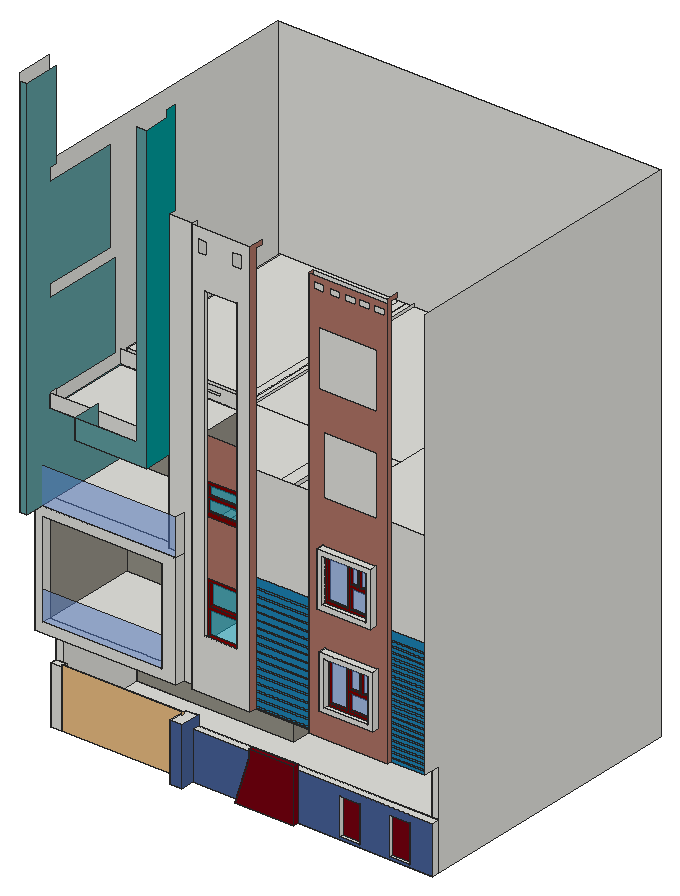
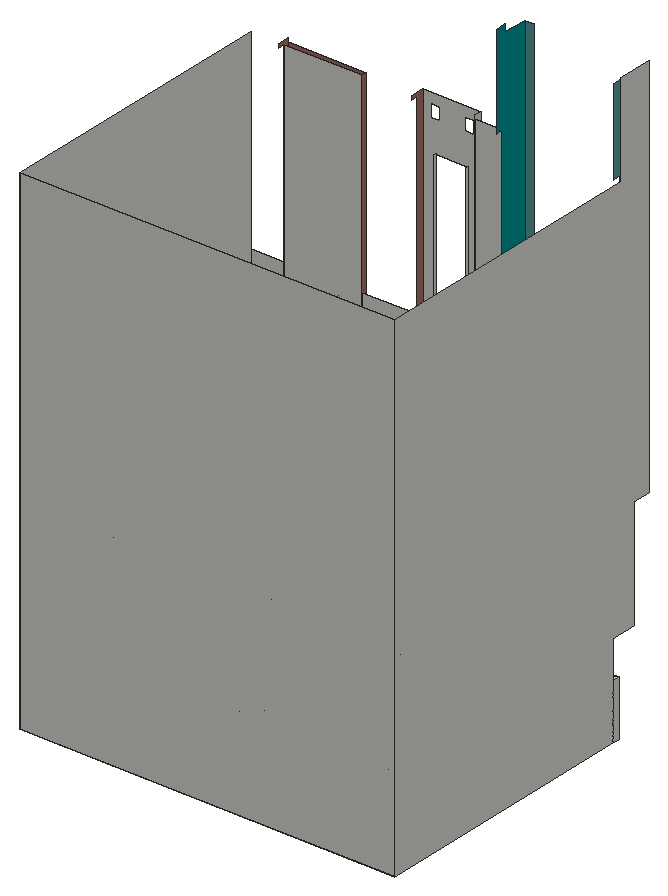
# SketchUp Ruby script. Lengths in inches.
U = 1.inch
M = Sketchup.active_model
def pt(a) = Geom::Point3d.new(a.map { |v| v * U })
def face(e, loops, mat)
  f = e.add_face(loops[0].map { |a| pt(a) })
  loops[1..].each { |l| e.add_face(l.map { |a| pt(a) }).erase! }
  f.material = f.back_material = mat if mat
  f
end
# faces: each face lists its corners as indices into pts; further lists are holes
def faces(e, pts, list, mat = nil) = list.each { |f| face(e, (f[0].is_a?(Array) ? f : [f]).map { |l| l.map { |i| pts[i] } }, mat) }
# xy, xz, yz: faces in a plane at the given z, y or x. An outline is a flat list of corners, or four numbers for a rectangle; further outlines are holes
def ring(l) = l.size == 4 ? [[l[0], l[1]], [l[2], l[1]], [l[2], l[3]], [l[0], l[3]]] : l.each_slice(2).to_a
def flat(e, list, mat, &to3) = list.each { |f| face(e, (f[0].is_a?(Array) ? f : [f]).map { |l| ring(l).map { |u, v| to3.(u, v) } }, mat) }
def xy(e, z, list, mat = nil) = flat(e, list, mat) { |x, y| [x, y, z] }
def xz(e, y, list, mat = nil) = flat(e, list, mat) { |x, z| [x, y, z] }
def yz(e, x, list, mat = nil) = flat(e, list, mat) { |y, z| [x, y, z] }
def lines(e, pts, list) = list.each { |a, b| e.add_line(pt(pts[a]), pt(pts[b])) }
# prism: a flat outline (further loops are holes) pulled along v
def prism(e, loops, v, mat = nil)
  f = face(e, loops, mat); d = Geom::Vector3d.new(v.map { |x| x * U })
  f.pushpull(f.normal.samedirection?(d) ? d.length : -d.length)
end
def box(e, o, s, mat = nil) = prism(e, [[o, [o[0] + s[0], o[1], o[2]], [o[0] + s[0], o[1] + s[1], o[2]], [o[0], o[1] + s[1], o[2]]]], [0, 0, s[2]], mat)
def at(x, y, z, deg = 0) = Geom::Transformation.translation(pt([x, y, z])) * Geom::Transformation.rotation(ORIGIN, Z_AXIS, deg.degrees)
def axes(o, x, y, z) = Geom::Transformation.new([*x, 0, *y, 0, *z, 0, *pt(o).to_a, 1])
def part(name) = M.definitions.add(name)
# library, detail: a bought-in or finely detailed component or shape, given as its bounding box
def library(name, o, s) = part(name).tap { |d| box(d.entities, o, s) }
def detail(e, o, s) = box(e.add_group.entities, o, s)
def put(e, d, t, mat = nil) = e.add_instance(d, t).tap { |i| i.material = mat if mat }
def group(e, t, mat = nil) = e.add_group.tap { |g| g.transformation = t; g.material = mat if mat }.entities
root = M.entities
M.materials.add("[0022_Maroon]").color = [128, 0, 0]
M.materials.add("[0081_CadetBlue]").color = [95, 158, 160]
M.materials.add("[0100_SteelBlue]").color = [29, 130, 180]
M.materials.add("[Color H07]").color = [0, 153, 153]
M.materials.add("[Formica Blue]").color = [71, 97, 152]
M.materials.add("[Formica Graystone]").color = [149, 146, 135]
M.materials.add("[Sketchy Siding Straight]").color = [119, 0, 16]
M.materials.add("[Stone Flagstone Ashlar]").color = [175, 116, 102]
M.materials.add("[Translucent Glass Blue]").color = [100, 149, 237]
M.materials["[Translucent Glass Blue]"].alpha = 0.5
M.materials.add("[Translucent Glass Tinted]").color = [8, 201, 241]
M.materials["[Translucent Glass Tinted]"].alpha = 0.48
c1 = library("gate (1)",[0,0,0],[171.26,1.97,78.74])
box(root,[9,163.25,173.75],[154.01,236.0625,120])
xy(root,41.75,[[164.3,31.6875,164.3,57.3125,360,57.3125,360,48.3125,312.21,48.3125,312.21,42.3125,238.26,42.3125,238.26,48.3125,179.85,48.3125,179.85,31.6875],[0,48.3125,13.95,57.3125],[360,48.3125,483.5625,57.3125],[0,57.3125,0,408.3125,360,408.3125,360,399.3125,9,399.3125,9,57.3125],[9,57.3125,474.5625,57.3125,474.5625,399.3125,207.375,399.3125,207.375,173.875,9,173.875],
  [474.5625,57.3125,474.5625,399.3125,360,399.3125,360,408.3125,483.5625,408.3125,483.5625,57.3125],[9,173.875,9,179.875,201.375,179.875,201.375,399.3125,207.375,399.3125,207.375,173.875],[9,179.875,201.375,399.3125]])
xy(root,44.78,[[365.45,48.3125,391.2,53],[428.88,48.3125,454.63,52.0625]])
xy(root,77.84,[[79.99,170.875,183.74,173.875]])
xy(root,78.43,[[21.52,170.875,59.52,173.875]])
xy(root,80.84,[[82.99,170.875,102.77,173.875],[106.875,170.875,180.74,173.875]],"[0022_Maroon]")
xy(root,81.43,[[24.52,170.875,56.52,173.875]],"[0022_Maroon]")
xy(root,91.78,[[365.45,48.3125,391.2,53],[428.88,48.3125,454.63,52.0625]])
xy(root,101.75,[[179.85,48.3125,483.5625,57.3125]])
xy(root,108.53,[[255.96,42.3125,312.21,48.3125]],"[Sketchy Siding Straight]")
xy(root,113.75,[[164.3,31.6875,179.85,57.3125],[0,48.3125,13.95,57.3125]])
xy(root,145.3,[[24.52,170.875,56.52,173.875]],"[0022_Maroon]")
xy(root,148.09,[[82.99,170.875,102.77,173.875],[106.875,170.875,180.74,173.875]],"[0022_Maroon]")
xy(root,148.3,[[21.52,170.875,59.52,173.875]])
xy(root,151.09,[[79.99,170.875,183.74,173.875]],"[0022_Maroon]")
xy(root,161.75,[[0,24,177.9375,36],[195.16,27,195.16,36,9,36,9,173.875,207.375,173.875,207.375,399.3125,474.5625,399.3125,474.5625,57.3125,483.5625,57.3125,483.5625,36,269.35,36,269.35,27],[341.01,30,440.77,36],[0,36,9,57.3125],[9,173.875,207.375,173.875,207.375,399.3125,201.375,399.3125,201.375,179.875,9,179.875],
  [9,179.875,201.375,399.3125]])
xy(root,173.75,[[9,24,160.01,36],[9,36,160.01,36,160.01,157.25,141.2,157.25,141.2,154.25,138.2,154.25,138.2,157.25,102.2,157.25,102.2,154.25,99.2,154.25,99.2,157.25,9,157.25],[99.2,154.25,102.2,157.25],[138.2,154.25,141.2,157.25]])
xy(root,197.9375,[[361.52,21,428.89,30]])
xy(root,203.9375,[[367.52,21,422.89,27]])
xy(root,206.9375,[[370.52,27,391.89,30],[395.21,27,419.89,30]],"[0022_Maroon]")
xy(root,218.125,[[18.2,154.25,89.13,157.25]])
xy(root,224.125,[[24.2,154.25,53.67,157.25],[57.96,154.25,83.13,157.25]],"[0022_Maroon]")
xy(root,227.89,[[395.21,27,419.89,30]],"[0022_Maroon]")
xy(root,228.47,[[211.91,27,253.16,27,253.16,30,250.36,30,250.36,32.1875,215.48,32.1875,215.48,30,211.91,30]],"[0022_Maroon]")
xy(root,231.625,[[395.21,27,407.55,30],[410.96,27,419.89,30]],"[0022_Maroon]")
xy(root,254.1875,[[57.96,154.25,83.13,157.25]],"[0022_Maroon]")
xy(root,256.3125,[[370.52,27,391.89,30],[395.21,27,407.55,30],[410.96,27,419.89,30]],"[0022_Maroon]")
xy(root,257.06,[[215.48,30,250.36,32.1875]],"[0022_Maroon]")
xy(root,257.75,[[102.2,154.25,138.2,157.25]],"[0022_Maroon]")
xy(root,259.3125,[[367.52,21,422.89,27]])
xy(root,259.36,[[57.96,154.25,83.13,157.25]],"[0022_Maroon]")
xy(root,260.75,[[99.2,154.25,141.2,157.25]],"[0022_Maroon]")
xy(root,261.21,[[215.48,30,250.36,35.4375]],"[0022_Maroon]")
xy(root,265.3125,[[361.52,21,428.89,30]])
xy(root,278.4375,[[24.2,154.25,53.67,157.25],[57.96,154.25,83.13,157.25]],"[0022_Maroon]")
xy(root,284.4375,[[18.2,154.25,89.13,157.25]],"[0022_Maroon]")
xy(root,289.07,[[215.48,30,250.36,35.4375]],"[0022_Maroon]")
xy(root,290.0625,[[9,36,160.01,157.25]],"[Formica Graystone]")
xy(root,293.75,[[9,24,160.01,36],[169.01,157.25,351,399.3125]])
xy(root,305.75,[[0,0,9,24],[9,23.22,9,24,177.9375,24],[9,24,177.9375,24,177.9375,36,160.01,36,160.01,45,9,45],[9,45,160.01,45,160.01,148.25,145.29,148.25,145.29,145.25,142.29,145.25,142.29,148.25,106.29,148.25,106.29,145.25,103.29,145.25,103.29,148.25,9,148.25],[103.29,145.25,106.29,148.25],
  [142.29,145.25,145.29,148.25],[160.01,148.25,169.01,157.25],[9,157.25,160.01,399.3125]])
xy(root,313.15,[[358.5,21,426.4375,30]])
xy(root,319.15,[[364.5,21,420.4375,27],[364.5,27,420.4375,30]])
xy(root,322.15,[[392.47,27,396.32,30]])
xy(root,322.15,[[367.5,27,392.47,30],[396.32,27,417.4375,30]],"[0022_Maroon]")
xy(root,337,[[25.5,145.25,96.62,148.25]])
xy(root,343,[[31.5,145.25,61.06,148.25],[64.41,145.25,90.62,148.25]],"[0022_Maroon]")
xy(root,347.12,[[396.32,27,417.4375,30]])
xy(root,350.93,[[396.32,27,405.07,30],[408.78,27,417.4375,30]],"[0022_Maroon]")
xy(root,368.85,[[214.81,30,250.11,31.875]],"[0022_Maroon]")
xy(root,372.09,[[367.5,27,392.47,30],[396.32,27,405.07,30],[408.78,27,417.4375,30]],"[0022_Maroon]")
xy(root,375.09,[[364.5,21,420.4375,27],[364.5,27,420.4375,30]])
xy(root,381.09,[[358.5,21,426.4375,30]])
xy(root,382.74,[[214.81,30,250.11,31.875]],"[0022_Maroon]")
xy(root,382.88,[[64.41,145.25,90.62,148.25]],"[0022_Maroon]")
xy(root,385.95,[[64.41,145.25,90.62,148.25]],"[0022_Maroon]")
xy(root,386.41,[[214.81,30,250.11,32.875]],"[0022_Maroon]")
xy(root,389.75,[[106.29,145.25,142.29,148.25]],"[0022_Maroon]")
xy(root,392.75,[[103.29,145.25,145.29,148.25]],"[0022_Maroon]")
xy(root,399,[[31.5,145.25,61.06,148.25],[64.41,145.25,90.62,148.25]],"[0022_Maroon]")
xy(root,399.35,[[214.81,30,250.11,32.875]])
xy(root,405,[[25.5,145.25,96.62,148.25]],"[0022_Maroon]")
xy(root,411.4375,[[9,36,160.01,148.25]])
xy(root,411.4375,[[69.02,0,160.01,36]],"[0081_CadetBlue]")
xy(root,425.75,[[160.01,148.25,169.01,157.25],[169.01,148.25,170.26,399.3125],[170.26,148.25,178.01,399.3125],[178.01,148.25,363.3125,399.3125],[9,157.25,160.01,399.3125],
  [160.01,157.25,169.01,399.3125]])
xz(root,0,[[0,305.75,9,794.55],[69.02,411.4375,160.01,411.4375,160.01,794.55,148.21,794.55,148.21,437.26,69.02,437.26]],"[0081_CadetBlue]")
xz(root,21,[[[361.52,197.9375,428.89,265.3125],[367.52,203.9375,422.89,259.3125]],[[358.5,313.15,426.4375,381.09],[364.5,319.15,420.4375,375.09]]])
xz(root,24,[[[0,161.75,177.9375,305.75],[9,173.75,160.01,293.75]]])
xz(root,24,[[9,173.75,160.01,211.88]],"[Translucent Glass Blue]")
xz(root,27,[[[195.16,161.75,269.35,688.75],[211.91,228.47,253.16,619.47],[203.22,659.36,215.03,675.93],[246.9,659.36,258.72,675.93]]])
xz(root,27,[[[367.52,203.9375,422.89,259.3125],[370.52,206.9375,391.89,256.3125],[395.21,206.9375,419.89,227.89],[395.21,231.625,407.55,256.3125],[410.96,231.625,419.89,256.3125]],[[364.5,319.15,420.4375,375.09],[367.5,322.15,367.5,372.09,392.47,372.09,392.47,322.15,396.32,322.15,396.32,347.12,417.4375,347.12,417.4375,322.15],[396.32,350.93,405.07,372.09],[408.78,350.93,417.4375,372.09]]],"[0022_Maroon]")
xz(root,30,[[[364.5,319.15,420.4375,375.09],[367.5,322.15,417.4375,322.15,417.4375,347.12,396.32,347.12,396.32,322.15,392.47,322.15,392.47,372.09,367.5,372.09],[396.32,350.93,405.07,372.09],[408.78,350.93,417.4375,372.09]]])
xz(root,30,[[[211.91,228.47,215.48,228.47,215.48,257.06,250.36,257.06,250.36,228.47,253.16,228.47,253.16,292.67,211.91,292.67],[215.48,261.21,250.36,289.07]],[[211.91,362.68,253.16,402.99],[214.81,368.85,250.11,382.74],[214.81,386.41,250.11,399.35]]],"[0022_Maroon]")
xz(root,30,[[[341.01,161.75,440.77,683.75],[353.5625,556.6,427.4375,626.6],[359.73,434.83,427.1,510.21],[358.5,313.15,426.4375,381.09],[361.52,197.9375,428.89,265.3125],[347.12,668.19,360.37,676.37],[367.68,668.19,380.93,676.37],[387.06,668.19,400.31,676.37],[404.68,668.19,417.93,676.37],[423.62,668.19,436.87,676.37]],[211.91,292.67,253.16,362.68],[211.91,402.99,253.16,454.38]],"[Stone Flagstone Ashlar]")
xz(root,30,[[370.52,206.9375,391.89,256.3125],[395.21,206.9375,419.89,227.89],[395.21,231.625,407.55,256.3125],[410.96,231.625,419.89,256.3125],[367.5,322.15,392.47,372.09],
  [396.32,322.15,417.4375,347.12],[396.32,350.93,405.07,372.09],[408.78,350.93,417.4375,372.09]],"[Translucent Glass Blue]")
xz(root,31.6875,[[164.3,41.75,179.85,113.75]],"[Formica Blue]")
xz(root,31.875,[[214.81,368.85,250.11,382.74]],"[Translucent Glass Tinted]")
xz(root,32.1875,[[215.48,228.47,250.36,257.06]],"[Translucent Glass Tinted]")
xz(root,32.875,[[214.81,386.41,250.11,399.35]],"[Translucent Glass Tinted]")
xz(root,35.4375,[[215.48,261.21,250.36,289.07]],"[Translucent Glass Tinted]")
xz(root,36,[[177.9375,161.75,195.16,161.75,195.16,683.75,160.01,683.75,160.01,305.75,177.9375,305.75],[341.01,161.75,440.77,683.75],[160.01,173.75,177.9375,293.375],[9,290.0625,160.01,293.375],[9,293.375,160.01,293.75],
  [269.35,311.26,341.01,432.69],[440.77,311.26,483.5625,433.25],[9,411.4375,69.02,428.75],[69.02,411.4375,160.01,428.75]])
xz(root,36,[[269.35,161.75,341.01,163.11],[440.77,161.75,483.5625,165.93],[269.35,163.11,341.01,165.14],[269.35,165.14,341.01,172.11],[440.77,165.93,483.5625,168.01],
  [440.77,168.01,483.5625,172.55],[269.35,172.11,341.01,174.14],[440.77,172.55,483.5625,174.63],[269.35,174.14,341.01,181.11],[440.77,174.63,483.5625,179.18],
  [440.77,179.18,483.5625,181.26],[269.35,181.11,341.01,183.14],[440.77,181.26,483.5625,185.8],[269.35,183.14,341.01,190.11],[440.77,185.8,483.5625,187.88],
  [440.77,187.88,483.5625,192.43],[269.35,190.11,341.01,192.14],[269.35,192.14,341.01,199.11],[440.77,192.43,483.5625,194.51],[440.77,194.51,483.5625,199.05],
  [440.77,199.05,483.5625,201.13],[269.35,199.11,341.01,201.14],[440.77,201.13,483.5625,205.68],[269.35,201.14,341.01,208.11],[440.77,205.68,483.5625,207.76],
  [440.77,207.76,483.5625,212.3],[269.35,208.11,341.01,210.14],[269.35,210.14,341.01,217.11],[440.77,212.3,483.5625,214.38],[440.77,214.38,483.5625,218.93],
  [269.35,217.11,341.01,219.14],[440.77,218.93,483.5625,221.01],[269.35,219.14,341.01,226.11],[440.77,221.01,483.5625,225.55],[440.77,225.55,483.5625,227.63],
  [269.35,226.11,341.01,228.14],[440.77,227.63,483.5625,232.18],[269.35,228.14,341.01,235.11],[440.77,232.18,483.5625,234.26],[440.77,234.26,483.5625,238.8],
  [269.35,235.11,341.01,237.14],[269.35,237.14,341.01,244.11],[440.77,238.8,483.5625,240.88],[440.77,240.88,483.5625,245.43],[269.35,244.11,341.01,246.14],
  [440.77,245.43,483.5625,247.51],[269.35,246.14,341.01,253.11],[440.77,247.51,483.5625,252.05],[440.77,252.05,483.5625,254.13],[269.35,253.11,341.01,255.14],
  [440.77,254.13,483.5625,258.68],[269.35,255.14,341.01,262.11],[440.77,258.68,483.5625,260.76],[440.77,260.76,483.5625,265.3],[269.35,262.11,341.01,264.14],
  [269.35,264.14,341.01,271.11],[440.77,265.3,483.5625,267.38],[440.77,267.38,483.5625,271.93],[269.35,271.11,341.01,273.14],[440.77,271.93,483.5625,274.01],
  [269.35,273.14,341.01,280.11],[440.77,274.01,483.5625,278.55],[440.77,278.55,483.5625,280.63],[269.35,280.11,341.01,282.14],[440.77,280.63,483.5625,285.18],
  [269.35,282.14,341.01,289.11],[440.77,285.18,483.5625,287.26],[440.77,287.26,483.5625,291.8],[269.35,289.11,341.01,291.14],[269.35,291.14,341.01,298.11],
  [440.77,291.8,483.5625,293.88],[440.77,293.88,483.5625,298.43],[269.35,298.11,341.01,300.14],[440.77,298.43,483.5625,300.51],[269.35,300.14,341.01,311.26],
  [440.77,300.51,483.5625,311.26]],"[0100_SteelBlue]")
xz(root,42.3125,[[238.26,41.75,312.21,41.75,312.21,108.53,255.96,108.53,255.96,98.97]],"[Sketchy Siding Straight]")
xz(root,48.3125,[[0,41.75,13.95,113.75],[255.96,98.97,312.21,101.75],[255.96,101.75,312.21,108.53]])
xz(root,48.3125,[[179.85,41.75,238.26,41.75,255.96,98.97,255.96,101.75,179.85,101.75],[[312.21,41.75,483.5625,101.75],[365.45,44.78,391.2,91.78],[428.88,44.78,454.63,91.78]]],"[Formica Blue]")
xz(root,52.0625,[[428.88,44.78,454.63,91.78]],"[Sketchy Siding Straight]")
xz(root,53,[[365.45,44.78,391.2,91.78]],"[Sketchy Siding Straight]")
xz(root,57.3125,[[0,41.75,9,101.75],[9,41.75,13.95,101.75],[164.3,41.75,360,101.75],[360,41.75,474.5625,101.75],[474.5625,41.75,483.5625,101.75],
  [0,101.75,9,113.75],[9,101.75,13.95,113.75],[164.3,101.75,179.85,113.75],[474.5625,101.75,483.5625,161.75],[0,113.75,9,161.75]])
xz(root,139.25,[[99.38,425.75,141.38,428.75]])
xz(root,145.25,[[103.29,305.75,106.29,305.75,106.29,389.75,142.29,389.75,142.29,305.75,145.29,305.75,145.29,392.75,103.29,392.75],[[25.5,337,96.62,405],[31.5,343,61.06,399],[64.41,343,90.62,382.88],[64.41,385.95,90.62,399]]],"[0022_Maroon]")
xz(root,148.25,[[103.29,302.75,145.29,305.75],[103.29,305.75,103.29,392.75,145.29,392.75,145.29,305.75,142.29,305.75,142.29,389.75,106.29,389.75,106.29,305.75],[160.01,305.75,169.01,425.75],[169.01,305.75,170.26,425.75],[[25.5,337,96.62,405],[31.5,343,61.06,399],[64.41,343,90.62,382.88],[64.41,385.95,90.62,399]],
  [9,411.4375,160.01,411.4375,160.01,425.75,178.01,425.75,178.01,428.75,9,428.75]])
xz(root,148.25,[[[9,305.75,103.29,305.75,103.29,392.75,145.29,392.75,145.29,305.75,160.01,305.75,160.01,411.4375,9,411.4375],[25.5,337,96.62,405]]],"[Formica Graystone]")
xz(root,148.25,[[106.29,305.75,142.29,389.75],[31.5,343,61.06,399],[64.41,343,90.62,382.88],[64.41,385.95,90.62,399]],"[Translucent Glass Blue]")
xz(root,154.25,[[99.2,173.75,102.2,173.75,102.2,257.75,138.2,257.75,138.2,173.75,141.2,173.75,141.2,260.75,99.2,260.75],[[18.2,218.125,89.13,284.4375],[24.2,224.125,53.67,278.4375],[57.96,224.125,83.13,254.1875],[57.96,259.36,83.13,278.4375]]],"[0022_Maroon]")
xz(root,157.25,[[99.2,170.75,141.2,173.75],[99.2,173.75,99.2,260.75,141.2,260.75,141.2,173.75,138.2,173.75,138.2,257.75,102.2,257.75,102.2,173.75],[[18.2,218.125,89.13,284.4375],[24.2,224.125,53.67,278.4375],[57.96,224.125,83.13,254.1875],[57.96,259.36,83.13,278.4375]],[9,290.0625,160.01,290.0625,160.01,293.75,169.01,293.75,169.01,305.75,9,305.75],[9,305.75,169.01,425.75]])
xz(root,157.25,[[[9,173.75,99.2,173.75,99.2,260.75,141.2,260.75,141.2,173.75,160.01,173.75,160.01,290.0625,9,290.0625],[18.2,218.125,89.13,284.4375]]],"[Formica Graystone]")
xz(root,157.25,[[102.2,173.75,138.2,257.75],[24.2,224.125,53.67,278.4375],[57.96,224.125,83.13,254.1875],[57.96,259.36,83.13,278.4375]],"[Translucent Glass Blue]")
xz(root,170.875,[[[79.99,77.84,183.74,151.09],[106.875,80.84,180.74,148.09],[82.99,80.84,102.77,148.09]],[[21.52,78.43,59.52,148.3],[24.52,81.43,56.52,145.3]]],"[0022_Maroon]")
xz(root,173.875,[[[79.99,77.84,183.74,151.09],[106.875,80.84,180.74,148.09],[82.99,80.84,102.77,148.09]],[[21.52,78.43,59.52,148.3],[24.52,81.43,56.52,145.3]]])
xz(root,173.875,[[[9,41.75,207.375,161.75],[79.99,77.84,183.74,151.09],[21.52,78.43,59.52,148.3]]],"[Formica Graystone]")
xz(root,173.875,[[82.99,80.84,102.77,148.09],[106.875,80.84,180.74,148.09],[24.52,81.43,56.52,145.3]],"[Translucent Glass Blue]")
xz(root,179.875,[[9,41.75,201.375,161.75]])
xz(root,399.3125,[[9,41.75,201.375,161.75],[201.375,41.75,207.375,161.75],[169.01,173.75,351,293.75]])
xz(root,399.3125,[[207.375,41.75,474.5625,161.75]],"[Formica Graystone]")
xz(root,408.3125,[[0,41.75,483.5625,683.75]])
yz(root,0,[[57.3125,41.75,57.3125,161.75,24,161.75,24,305.75,0,305.75,0,803.75,45,803.75,45,683.75,408.3125,683.75,408.3125,41.75],[48.3125,41.75,57.3125,113.75]])
yz(root,9,[[57.3125,41.75,173.875,161.75],[173.875,41.75,179.875,161.75],[179.875,41.75,399.3125,161.75],[24,173.75,36,293.75],[157.25,305.75,399.3125,425.75],
  [36,411.4375,45,428.75]])
yz(root,9,[[0,305.75,148.25,305.75,148.25,411.4375,36,411.4375,36,428.75,139.25,428.75,139.25,535.625,36,535.625,36,551.75,130.25,551.75,130.25,667.8125,36,667.8125,36,683.75,45,683.75,45,794.55,0,794.55]],"[0081_CadetBlue]")
yz(root,9,[[36,173.75,157.25,290.0625]],"[Formica Graystone]")
yz(root,13.95,[[48.3125,41.75,57.3125,113.75]])
yz(root,18.2,[[154.25,218.125,157.25,284.4375]])
yz(root,21.52,[[170.875,78.43,173.875,148.3]],"[0022_Maroon]")
yz(root,24.2,[[154.25,224.125,157.25,278.4375]],"[0022_Maroon]")
yz(root,24.52,[[170.875,81.43,173.875,145.3]],"[0022_Maroon]")
yz(root,25.5,[[145.25,337,148.25,405]],"[0022_Maroon]")
yz(root,31.5,[[145.25,343,148.25,399]],"[0022_Maroon]")
yz(root,53.67,[[154.25,224.125,157.25,278.4375]],"[0022_Maroon]")
yz(root,56.52,[[170.875,81.43,173.875,145.3]],"[0022_Maroon]")
yz(root,57.96,[[154.25,224.125,157.25,254.1875],[154.25,259.36,157.25,278.4375]],"[0022_Maroon]")
yz(root,59.52,[[170.875,78.43,173.875,148.3]],"[0022_Maroon]")
yz(root,61.06,[[145.25,343,148.25,399]],"[0022_Maroon]")
yz(root,64.41,[[145.25,343,148.25,382.88],[145.25,385.95,148.25,399]],"[0022_Maroon]")
yz(root,69.02,[[0,411.4375,36,437.26]],"[0081_CadetBlue]")
yz(root,79.99,[[170.875,77.84,173.875,151.09]],"[0022_Maroon]")
yz(root,82.99,[[170.875,80.84,173.875,148.09]],"[0022_Maroon]")
yz(root,83.13,[[154.25,224.125,157.25,254.1875],[154.25,259.36,157.25,278.4375]],"[0022_Maroon]")
yz(root,89.13,[[154.25,218.125,157.25,284.4375]],"[0022_Maroon]")
yz(root,90.62,[[145.25,343,148.25,382.88],[145.25,385.95,148.25,399]],"[0022_Maroon]")
yz(root,96.62,[[145.25,337,148.25,405]],"[0022_Maroon]")
yz(root,99.2,[[154.25,173.75,157.25,260.75]],"[0022_Maroon]")
yz(root,102.2,[[154.25,173.75,157.25,257.75]],"[0022_Maroon]")
yz(root,102.77,[[170.875,80.84,173.875,148.09]],"[0022_Maroon]")
yz(root,103.29,[[145.25,305.75,148.25,392.75]],"[0022_Maroon]")
yz(root,106.29,[[145.25,305.75,148.25,389.75]],"[0022_Maroon]")
yz(root,106.875,[[170.875,80.84,173.875,148.09]],"[0022_Maroon]")
yz(root,138.2,[[154.25,173.75,157.25,257.75]],"[0022_Maroon]")
yz(root,141.2,[[154.25,173.75,157.25,260.75]])
yz(root,142.29,[[145.25,305.75,148.25,389.75]],"[0022_Maroon]")
yz(root,145.29,[[145.25,305.75,148.25,392.75]])
yz(root,160.01,[[24,173.75,36,293.375],[24,293.375,36,293.75]])
yz(root,160.01,[[0,411.4375,36,411.4375,36,683.75,45,683.75,45,803.75,31.4375,803.75,31.4375,794.55,0,794.55]],"[Color H07]")
yz(root,160.01,[[36,173.75,157.25,290.0625],[36,305.75,148.25,411.4375]],"[Formica Graystone]")
yz(root,164.3,[[31.6875,41.75,57.3125,113.75]])
yz(root,177.9375,[[24,161.75,36,305.75],[24,305.75,36,352.22]])
yz(root,178.01,[[148.25,425.75,399.3125,428.75]])
yz(root,179.85,[[31.6875,41.75,48.3125,41.75,48.3125,101.75,57.3125,101.75,57.3125,113.75,31.6875,113.75]],"[Formica Blue]")
yz(root,180.74,[[170.875,80.84,173.875,148.09]],"[0022_Maroon]")
yz(root,183.74,[[170.875,77.84,173.875,151.09]],"[0022_Maroon]")
yz(root,195.16,[[27,161.75,36,688.75]])
yz(root,201.375,[[179.875,41.75,399.3125,161.75]])
yz(root,207.375,[[173.875,41.75,399.3125,161.75]],"[Formica Graystone]")
yz(root,211.91,[[27,228.47,30,619.47]])
yz(root,214.81,[[30,368.85,31.875,382.74],[30,386.41,32.875,399.35]],"[0022_Maroon]")
yz(root,215.48,[[30,228.47,32.1875,257.06],[30,261.21,35.4375,289.07]],"[0022_Maroon]")
yz(root,250.11,[[30,368.85,31.875,382.74],[30,386.41,32.875,399.35]],"[0022_Maroon]")
yz(root,250.36,[[30,228.47,32.1875,257.06],[30,261.21,35.4375,289.07]],"[0022_Maroon]")
yz(root,253.16,[[27,228.47,30,619.47]])
yz(root,255.96,[[42.3125,98.97,48.3125,108.53]],"[Sketchy Siding Straight]")
yz(root,269.35,[[27,161.75,36,161.75,36,683.75,45,683.75,45,688.75,27,688.75]],"[Stone Flagstone Ashlar]")
yz(root,312.21,[[42.3125,41.75,48.3125,108.53]],"[Sketchy Siding Straight]")
yz(root,341.01,[[30,161.75,36,683.75]],"[Stone Flagstone Ashlar]")
yz(root,351,[[66.3125,293.75,399.3125,301.4375]])
yz(root,358.5,[[21,313.15,30,381.09]])
yz(root,361.52,[[21,197.9375,30,265.3125]])
yz(root,364.5,[[21,319.15,27,375.09],[27,319.15,30,375.09]])
yz(root,365.45,[[48.3125,44.78,53,91.78]])
yz(root,367.5,[[27,322.15,30,372.09]],"[0022_Maroon]")
yz(root,367.52,[[21,203.9375,27,259.3125]])
yz(root,370.52,[[27,206.9375,30,256.3125]],"[0022_Maroon]")
yz(root,391.2,[[48.3125,44.78,53,91.78]])
yz(root,391.89,[[27,206.9375,30,256.3125]],"[0022_Maroon]")
yz(root,392.47,[[27,322.15,30,372.09]],"[0022_Maroon]")
yz(root,395.21,[[27,206.9375,30,227.89],[27,231.625,30,256.3125]],"[0022_Maroon]")
yz(root,396.32,[[27,322.15,30,347.12],[27,350.93,30,372.09]],"[0022_Maroon]")
yz(root,405.07,[[27,350.93,30,372.09]],"[0022_Maroon]")
yz(root,407.55,[[27,231.625,30,256.3125]],"[0022_Maroon]")
yz(root,408.78,[[27,350.93,30,372.09]],"[0022_Maroon]")
yz(root,410.96,[[27,231.625,30,256.3125]],"[0022_Maroon]")
yz(root,417.4375,[[27,322.15,30,347.12],[27,350.93,30,372.09]],"[0022_Maroon]")
yz(root,419.89,[[27,206.9375,30,227.89],[27,231.625,30,256.3125]],"[0022_Maroon]")
yz(root,420.4375,[[21,319.15,27,375.09],[27,319.15,30,375.09]])
yz(root,422.89,[[21,203.9375,27,259.3125]])
yz(root,426.4375,[[21,313.15,30,381.09]])
yz(root,428.88,[[48.3125,44.78,52.0625,91.78]])
yz(root,428.89,[[21,197.9375,30,265.3125]])
yz(root,440.77,[[30,161.75,36,161.75,36,683.75,45,683.75,45,688.75,30,688.75]],"[Stone Flagstone Ashlar]")
yz(root,454.63,[[48.3125,44.78,52.0625,91.78]])
yz(root,474.5625,[[57.3125,41.75,399.3125,161.75]],"[Formica Graystone]")
yz(root,483.5625,[[57.3125,41.75,408.3125,41.75,408.3125,683.75,36,683.75,36,161.75,57.3125,161.75],[48.3125,41.75,57.3125,101.75]])
p = [[255.96,48.3125,98.97],[238.26,48.3125,41.75],[238.26,42.3125,41.75],[255.96,42.3125,98.97],[9,23.22,305.75],[177.9375,24,305.75],
  [177.9375,24,352.22],[9,23.22,352.22],[201.375,399.3125,161.75],[201.375,408.3125,161.75],[9,399.3125,161.75],[9,408.3125,161.75],
  [351,36,173.75],[351,157.25,173.75],[160.01,157.25,173.75],[169.01,399.3125,173.75],[169.01,408.3125,173.75],[9,157.25,293.75],
  [9,163.25,293.75],[9,399.3125,293.75],[0,399.3125,293.75],[351,66.3125,301.4375],[351,36,301.4375],[351,399.3125,301.4375],
  [169.01,399.3125,301.4375],[363.3125,148.25,305.75],[363.3125,36,305.75],[169.01,399.3125,305.75],[160.01,399.3125,305.75],[363.3125,399.3125,425.75],
  [372.3125,399.3125,425.75],[170.26,148.25,305.75],[351,399.3125,173.75],[170.26,36,305.75],[363.3125,45,425.75],[363.3125,148.25,425.75],
  [363.3125,408.3125,305.75],[160.01,408.3125,305.75]]
faces(root,p,[[0,1,2,3]],"[Sketchy Siding Straight]")
faces(root,p,[[4,5,6,7]],"[Translucent Glass Blue]")
lines(root,p,[[8,9],[10,11],[12,13],[13,14],[15,16],[17,18],[19,20],[21,22],[23,24],[25,26],[27,28],[29,30],
  [25,31],[13,32],[33,31],[34,35],[25,36],[28,37]])
put(root,c1,axes([13.95,48.53,41.75],[0.89,0,0],[0,0.89,0],[0,0,0.94411]))
